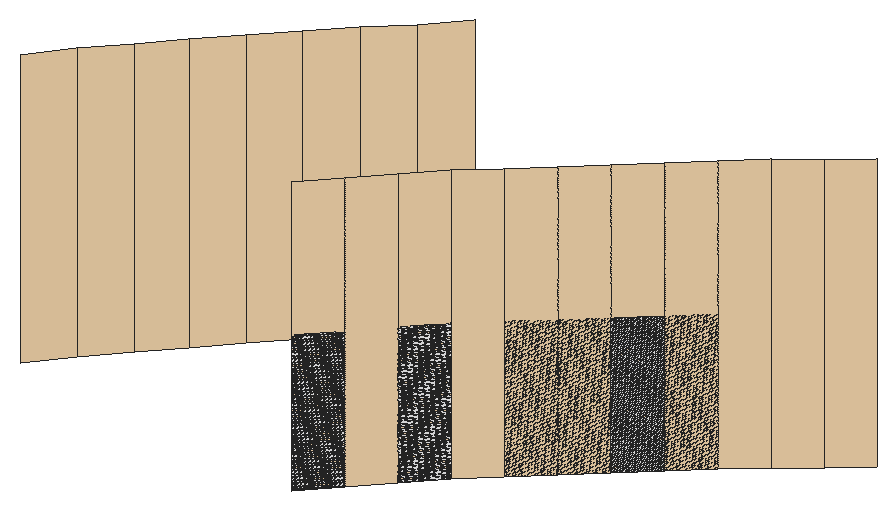
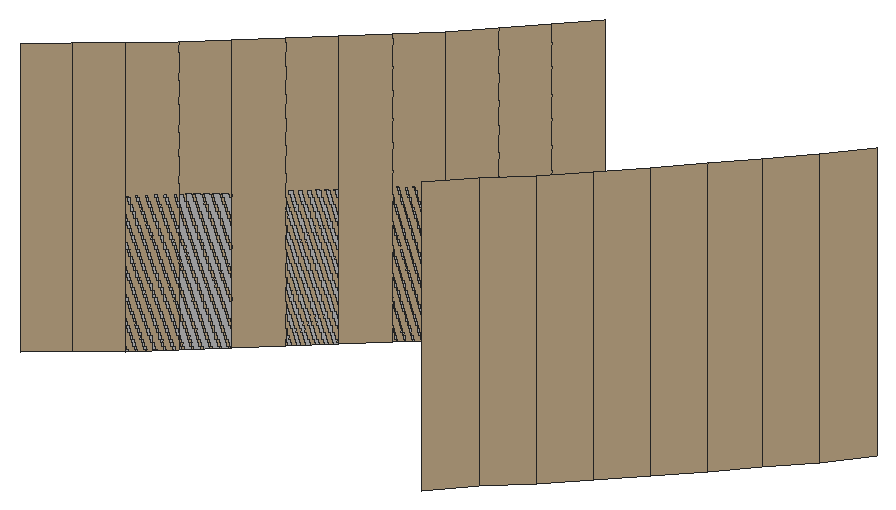
# SketchUp Ruby script. Lengths in inches.
U = 1.inch
M = Sketchup.active_model
def pt(a) = Geom::Point3d.new(a.map { |v| v * U })
def face(e, loops, mat)
  f = e.add_face(loops[0].map { |a| pt(a) })
  loops[1..].each { |l| e.add_face(l.map { |a| pt(a) }).erase! }
  f.material = f.back_material = mat if mat
  f
end
# faces: each face lists its corners as indices into pts; further lists are holes
def faces(e, pts, list, mat = nil) = list.each { |f| face(e, (f[0].is_a?(Array) ? f : [f]).map { |l| l.map { |i| pts[i] } }, mat) }
# xy, xz, yz: faces in a plane at the given z, y or x. An outline is a flat list of corners, or four numbers for a rectangle; further outlines are holes
def ring(l) = l.size == 4 ? [[l[0], l[1]], [l[2], l[1]], [l[2], l[3]], [l[0], l[3]]] : l.each_slice(2).to_a
def flat(e, list, mat, &to3) = list.each { |f| face(e, (f[0].is_a?(Array) ? f : [f]).map { |l| ring(l).map { |u, v| to3.(u, v) } }, mat) }
def xy(e, z, list, mat = nil) = flat(e, list, mat) { |x, y| [x, y, z] }
def xz(e, y, list, mat = nil) = flat(e, list, mat) { |x, z| [x, y, z] }
def yz(e, x, list, mat = nil) = flat(e, list, mat) { |y, z| [x, y, z] }
def lines(e, pts, list) = list.each { |a, b| e.add_line(pt(pts[a]), pt(pts[b])) }
# prism: a flat outline (further loops are holes) pulled along v
def prism(e, loops, v, mat = nil)
  f = face(e, loops, mat); d = Geom::Vector3d.new(v.map { |x| x * U })
  f.pushpull(f.normal.samedirection?(d) ? d.length : -d.length)
end
def box(e, o, s, mat = nil) = prism(e, [[o, [o[0] + s[0], o[1], o[2]], [o[0] + s[0], o[1] + s[1], o[2]], [o[0], o[1] + s[1], o[2]]]], [0, 0, s[2]], mat)
def at(x, y, z, deg = 0) = Geom::Transformation.translation(pt([x, y, z])) * Geom::Transformation.rotation(ORIGIN, Z_AXIS, deg.degrees)
def axes(o, x, y, z) = Geom::Transformation.new([*x, 0, *y, 0, *z, 0, *pt(o).to_a, 1])
def part(name) = M.definitions.add(name)
# library, detail: a bought-in or finely detailed component or shape, given as its bounding box
def library(name, o, s) = part(name).tap { |d| box(d.entities, o, s) }
def detail(e, o, s) = box(e.add_group.entities, o, s)
def put(e, d, t, mat = nil) = e.add_instance(d, t).tap { |i| i.material = mat if mat }
def group(e, t, mat = nil) = e.add_group.tap { |g| g.transformation = t; g.material = mat if mat }.entities
root = M.entities
M.materials.add("False Ceiling Light").color = [254, 223, 179]
M.materials.add("[Quartz Light Grey]").color = [251, 251, 252]
p = [[47.09,213.16,115.32],[47.21,213.29,115.32],[47.21,213.29,116.49],[47.09,213.16,116.49],[47.21,213.29,115.32],[47.09,213.16,115.32],
  [47.09,213.16,115.91],[47.21,213.29,115.91],[45.97,213.42,115.32],[45.85,213.27,115.32],[45.85,213.27,116.49],[45.97,213.42,116.49],
  [47.33,213.42,115.32],[47.33,213.42,116.49],[47.33,213.42,115.32],[47.33,213.42,115.91],[46.1,213.5625,115.32],[46.1,213.5625,116.49],
  [47.45,213.55,115.32],[47.45,213.55,116.49],[47.45,213.55,115.32],[47.45,213.55,115.91],[47.58,213.67,115.32],[47.58,213.67,116.49],
  [47.58,213.67,115.32],[47.58,213.67,115.91],[46.22,213.7,115.32],[46.22,213.7,116.49],[46.35,213.84,115.32],[46.35,213.84,116.49],
  [47.71,213.79,115.32],[47.71,213.79,116.49],[47.71,213.79,115.32],[47.71,213.79,115.91],[46.48,213.98,115.32],[46.48,213.98,116.49],
  [47.84,213.91,115.32],[47.84,213.91,116.49],[47.84,213.91,115.32],[47.84,213.91,115.91],[47.97,214.03,115.32],[47.97,214.03,116.49],
  [47.97,214.03,115.32],[47.97,214.03,115.91],[46.61,214.12,115.32],[46.61,214.12,116.49],[48.1,214.15,115.32],[48.1,214.15,116.49],
  [48.1,214.15,115.32],[48.1,214.15,115.91],[46.75,214.25,115.32],[46.75,214.25,116.49],[48.23,214.27,115.32],[48.23,214.27,116.49],
  [48.23,214.27,115.32],[48.23,214.27,115.91],[46.88,214.39,115.32],[46.88,214.39,116.49],[48.37,214.38,115.32],[48.37,214.38,116.49],
  [48.37,214.38,115.32],[48.37,214.38,115.91],[48.5,214.49,115.32],[48.5,214.49,116.49]]
faces(root,p,[[0,1,2,3],[8,9,10,11],[1,12,13,2],[16,8,11,17],[12,18,19,13],[18,22,23,19],[26,16,17,27],[28,26,27,29],
  [22,30,31,23],[34,28,29,35],[30,36,37,31],[36,40,41,37],[44,34,35,45],[40,46,47,41],[50,44,45,51],[46,52,53,47],
  [56,50,51,57],[52,58,59,53],[58,62,63,59]],"False Ceiling Light")
faces(root,p,[[4,5,6,7],[14,4,7,15],[20,14,15,21],[24,20,21,25],[32,24,25,33],[38,32,33,39],[42,38,39,43],[48,42,43,49],
  [54,48,49,55],[60,54,55,61]],"[Quartz Light Grey]")
